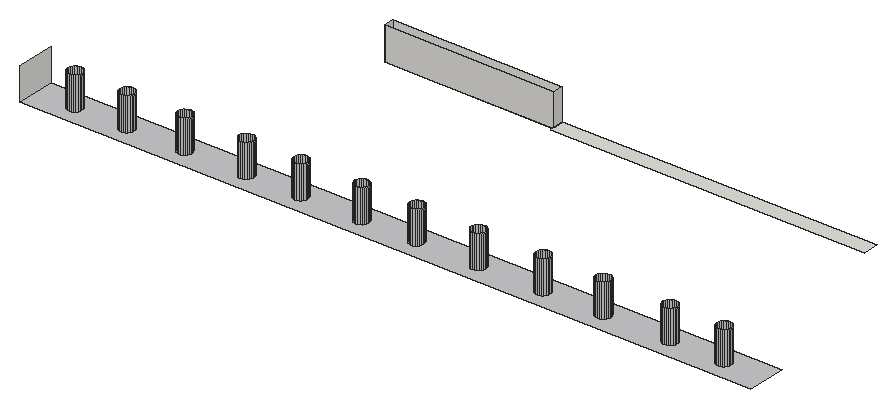
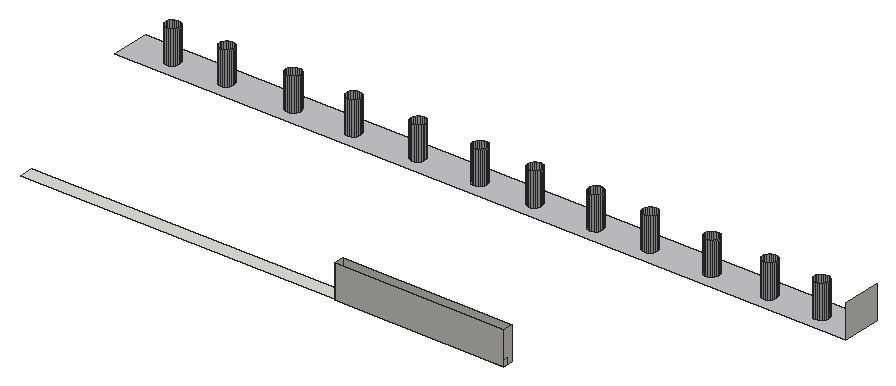
# SketchUp Ruby script. Lengths in inches.
U = 1.inch
M = Sketchup.active_model
def pt(a) = Geom::Point3d.new(a.map { |v| v * U })
def face(e, loops, mat)
  f = e.add_face(loops[0].map { |a| pt(a) })
  loops[1..].each { |l| e.add_face(l.map { |a| pt(a) }).erase! }
  f.material = f.back_material = mat if mat
  f
end
# faces: each face lists its corners as indices into pts; further lists are holes
def faces(e, pts, list, mat = nil) = list.each { |f| face(e, (f[0].is_a?(Array) ? f : [f]).map { |l| l.map { |i| pts[i] } }, mat) }
# xy, xz, yz: faces in a plane at the given z, y or x. An outline is a flat list of corners, or four numbers for a rectangle; further outlines are holes
def ring(l) = l.size == 4 ? [[l[0], l[1]], [l[2], l[1]], [l[2], l[3]], [l[0], l[3]]] : l.each_slice(2).to_a
def flat(e, list, mat, &to3) = list.each { |f| face(e, (f[0].is_a?(Array) ? f : [f]).map { |l| ring(l).map { |u, v| to3.(u, v) } }, mat) }
def xy(e, z, list, mat = nil) = flat(e, list, mat) { |x, y| [x, y, z] }
def xz(e, y, list, mat = nil) = flat(e, list, mat) { |x, z| [x, y, z] }
def yz(e, x, list, mat = nil) = flat(e, list, mat) { |y, z| [x, y, z] }
def lines(e, pts, list) = list.each { |a, b| e.add_line(pt(pts[a]), pt(pts[b])) }
# prism: a flat outline (further loops are holes) pulled along v
def prism(e, loops, v, mat = nil)
  f = face(e, loops, mat); d = Geom::Vector3d.new(v.map { |x| x * U })
  f.pushpull(f.normal.samedirection?(d) ? d.length : -d.length)
end
def box(e, o, s, mat = nil) = prism(e, [[o, [o[0] + s[0], o[1], o[2]], [o[0] + s[0], o[1] + s[1], o[2]], [o[0], o[1] + s[1], o[2]]]], [0, 0, s[2]], mat)
def at(x, y, z, deg = 0) = Geom::Transformation.translation(pt([x, y, z])) * Geom::Transformation.rotation(ORIGIN, Z_AXIS, deg.degrees)
def axes(o, x, y, z) = Geom::Transformation.new([*x, 0, *y, 0, *z, 0, *pt(o).to_a, 1])
def part(name) = M.definitions.add(name)
# library, detail: a bought-in or finely detailed component or shape, given as its bounding box
def library(name, o, s) = part(name).tap { |d| box(d.entities, o, s) }
def detail(e, o, s) = box(e.add_group.entities, o, s)
def put(e, d, t, mat = nil) = e.add_instance(d, t).tap { |i| i.material = mat if mat }
def group(e, t, mat = nil) = e.add_group.tap { |g| g.transformation = t; g.material = mat if mat }.entities
root = M.entities
M.materials.add("[Polished Concrete New]").color = [200, 200, 203]
M.materials.add("[Terrazzo Tile Accent]").color = [224, 221, 217]
xy(root,116.26,[[461.1,311.53,526.2,315.41]],"[Terrazzo Tile Accent]")
xy(root,116.34,[[406,228.82,405.29,228.92,404.625,229.19,404.06,229.63,403.62,230.2,403.34,230.86,403.25,231.57,403.34,232.29,403.62,232.95,404.06,233.52,404.625,233.96,405.29,234.23,406,234.32,406.71,234.23,407.375,233.96,407.94,233.52,408.38,232.95,408.66,232.29,408.75,231.57,408.66,230.86,408.38,230.2,407.94,229.63,407.375,229.19,406.71,228.92],[426,228.82,425.29,228.92,424.625,229.19,424.06,229.63,423.62,230.2,423.34,230.86,423.25,231.57,423.34,232.29,423.62,232.95,424.06,233.52,424.625,233.96,425.29,234.23,426,234.32,426.71,234.23,427.375,233.96,427.94,233.52,428.38,232.95,428.66,232.29,428.75,231.57,428.66,230.86,428.38,230.2,427.94,229.63,427.375,229.19,426.71,228.92],[448.1875,228.82,447.48,228.92,446.8125,229.19,446.24,229.63,445.81,230.2,445.53,230.86,445.4375,231.57,445.53,232.29,445.81,232.95,446.24,233.52,446.8125,233.96,447.48,234.23,448.1875,234.32,448.9,234.23,449.5625,233.96,450.13,233.52,450.57,232.95,450.84,232.29,450.9375,231.57,450.84,230.86,450.57,230.2,450.13,229.63,449.5625,229.19,448.9,228.92],[471.875,228.82,471.16,228.92,470.5,229.19,469.93,229.63,469.49,230.2,469.22,230.86,469.125,231.57,469.22,232.29,469.49,232.95,469.93,233.52,470.5,233.96,471.16,234.23,471.875,234.32,472.59,234.23,473.25,233.96,473.82,233.52,474.26,232.95,474.53,232.29,474.625,231.57,474.53,230.86,474.26,230.2,473.82,229.63,473.25,229.19,472.59,228.92],[492.8125,228.82,492.1,228.92,491.4375,229.19,490.87,229.63,490.43,230.2,490.16,230.86,490.0625,231.57,490.16,232.29,490.43,232.95,490.87,233.52,491.4375,233.96,492.1,234.23,492.8125,234.32,493.52,234.23,494.1875,233.96,494.76,233.52,495.19,232.95,495.47,232.29,495.5625,231.57,495.47,230.86,495.19,230.2,494.76,229.63,494.1875,229.19,493.52,228.92],
  [516.1875,228.82,515.48,228.92,514.8125,229.19,514.24,229.63,513.81,230.2,513.53,230.86,513.4375,231.57,513.53,232.29,513.81,232.95,514.24,233.52,514.8125,233.96,515.48,234.23,516.1875,234.32,516.9,234.23,517.5625,233.96,518.13,233.52,518.57,232.95,518.84,232.29,518.9375,231.57,518.84,230.86,518.57,230.2,518.13,229.63,517.5625,229.19,516.9,228.92],[537.375,228.82,536.66,228.92,536,229.19,535.43,229.63,534.99,230.2,534.72,230.86,534.625,231.57,534.72,232.29,534.99,232.95,535.43,233.52,536,233.96,536.66,234.23,537.375,234.32,538.09,234.23,538.75,233.96,539.32,233.52,539.76,232.95,540.03,232.29,540.125,231.57,540.03,230.86,539.76,230.2,539.32,229.63,538.75,229.19,538.09,228.92],[561.125,228.82,560.41,228.92,559.75,229.19,559.18,229.63,558.74,230.2,558.47,230.86,558.375,231.57,558.47,232.29,558.74,232.95,559.18,233.52,559.75,233.96,560.41,234.23,561.125,234.32,561.84,234.23,562.5,233.96,563.07,233.52,563.51,232.95,563.78,232.29,563.875,231.57,563.78,230.86,563.51,230.2,563.07,229.63,562.5,229.19,561.84,228.92],[585.9375,228.82,585.23,228.92,584.5625,229.19,583.99,229.63,583.56,230.2,583.28,230.86,583.1875,231.57,583.28,232.29,583.56,232.95,583.99,233.52,584.5625,233.96,585.23,234.23,585.9375,234.32,586.65,234.23,587.3125,233.96,587.88,233.52,588.32,232.95,588.59,232.29,588.6875,231.57,588.59,230.86,588.32,230.2,587.88,229.63,587.3125,229.19,586.65,228.92],[609.0625,228.82,608.35,228.92,607.6875,229.19,607.12,229.63,606.68,230.2,606.41,230.86,606.3125,231.57,606.41,232.29,606.68,232.95,607.12,233.52,607.6875,233.96,608.35,234.23,609.0625,234.32,609.77,234.23,610.4375,233.96,611.01,233.52,611.44,232.95,611.72,232.29,611.8125,231.57,611.72,230.86,611.44,230.2,611.01,229.63,610.4375,229.19,609.77,228.92],
  [634.75,228.82,634.04,228.92,633.375,229.19,632.81,229.63,632.37,230.2,632.09,230.86,632,231.57,632.09,232.29,632.37,232.95,632.81,233.52,633.375,233.96,634.04,234.23,634.75,234.32,635.46,234.23,636.125,233.96,636.69,233.52,637.13,232.95,637.41,232.29,637.5,231.57,637.41,230.86,637.13,230.2,636.69,229.63,636.125,229.19,635.46,228.92],[655.5,228.82,654.79,228.92,654.125,229.19,653.56,229.63,653.12,230.2,652.84,230.86,652.75,231.57,652.84,232.29,653.12,232.95,653.56,233.52,654.125,233.96,654.79,234.23,655.5,234.32,656.21,234.23,656.875,233.96,657.44,233.52,657.88,232.95,658.16,232.29,658.25,231.57,658.16,230.86,657.88,230.2,657.44,229.63,656.875,229.19,656.21,228.92]])
xy(root,116.34,[[[391.12,223.85,671.95,238.73],[655.5,228.82,654.79,228.92,654.125,229.19,653.56,229.63,653.12,230.2,652.84,230.86,652.75,231.57,652.84,232.29,653.12,232.95,653.56,233.52,654.125,233.96,654.79,234.23,655.5,234.32,656.21,234.23,656.875,233.96,657.44,233.52,657.88,232.95,658.16,232.29,658.25,231.57,658.16,230.86,657.88,230.2,657.44,229.63,656.875,229.19,656.21,228.92],[426,228.82,425.29,228.92,424.625,229.19,424.06,229.63,423.62,230.2,423.34,230.86,423.25,231.57,423.34,232.29,423.62,232.95,424.06,233.52,424.625,233.96,425.29,234.23,426,234.32,426.71,234.23,427.375,233.96,427.94,233.52,428.38,232.95,428.66,232.29,428.75,231.57,428.66,230.86,428.38,230.2,427.94,229.63,427.375,229.19,426.71,228.92],[634.75,228.82,634.04,228.92,633.375,229.19,632.81,229.63,632.37,230.2,632.09,230.86,632,231.57,632.09,232.29,632.37,232.95,632.81,233.52,633.375,233.96,634.04,234.23,634.75,234.32,635.46,234.23,636.125,233.96,636.69,233.52,637.13,232.95,637.41,232.29,637.5,231.57,637.41,230.86,637.13,230.2,636.69,229.63,636.125,229.19,635.46,228.92],[448.1875,228.82,447.48,228.92,446.8125,229.19,446.24,229.63,445.81,230.2,445.53,230.86,445.4375,231.57,445.53,232.29,445.81,232.95,446.24,233.52,446.8125,233.96,447.48,234.23,448.1875,234.32,448.9,234.23,449.5625,233.96,450.13,233.52,450.57,232.95,450.84,232.29,450.9375,231.57,450.84,230.86,450.57,230.2,450.13,229.63,449.5625,229.19,448.9,228.92],[609.0625,228.82,608.35,228.92,607.6875,229.19,607.12,229.63,606.68,230.2,606.41,230.86,606.3125,231.57,606.41,232.29,606.68,232.95,607.12,233.52,607.6875,233.96,608.35,234.23,609.0625,234.32,609.77,234.23,610.4375,233.96,611.01,233.52,611.44,232.95,611.72,232.29,611.8125,231.57,611.72,230.86,611.44,230.2,611.01,229.63,610.4375,229.19,609.77,228.92],[471.875,228.82,471.16,228.92,470.5,229.19,469.93,229.63,469.49,230.2,469.22,230.86,469.125,231.57,469.22,232.29,469.49,232.95,469.93,233.52,470.5,233.96,471.16,234.23,471.875,234.32,472.59,234.23,473.25,233.96,473.82,233.52,474.26,232.95,474.53,232.29,474.625,231.57,474.53,230.86,474.26,230.2,473.82,229.63,473.25,229.19,472.59,228.92],[585.9375,228.82,585.23,228.92,584.5625,229.19,583.99,229.63,583.56,230.2,583.28,230.86,583.1875,231.57,583.28,232.29,583.56,232.95,583.99,233.52,584.5625,233.96,585.23,234.23,585.9375,234.32,586.65,234.23,587.3125,233.96,587.88,233.52,588.32,232.95,588.59,232.29,588.6875,231.57,588.59,230.86,588.32,230.2,587.88,229.63,587.3125,229.19,586.65,228.92],[492.8125,228.82,492.1,228.92,491.4375,229.19,490.87,229.63,490.43,230.2,490.16,230.86,490.0625,231.57,490.16,232.29,490.43,232.95,490.87,233.52,491.4375,233.96,492.1,234.23,492.8125,234.32,493.52,234.23,494.1875,233.96,494.76,233.52,495.19,232.95,495.47,232.29,495.5625,231.57,495.47,230.86,495.19,230.2,494.76,229.63,494.1875,229.19,493.52,228.92],[561.125,228.82,560.41,228.92,559.75,229.19,559.18,229.63,558.74,230.2,558.47,230.86,558.375,231.57,558.47,232.29,558.74,232.95,559.18,233.52,559.75,233.96,560.41,234.23,561.125,234.32,561.84,234.23,562.5,233.96,563.07,233.52,563.51,232.95,563.78,232.29,563.875,231.57,563.78,230.86,563.51,230.2,563.07,229.63,562.5,229.19,561.84,228.92],[516.1875,228.82,515.48,228.92,514.8125,229.19,514.24,229.63,513.81,230.2,513.53,230.86,513.4375,231.57,513.53,232.29,513.81,232.95,514.24,233.52,514.8125,233.96,515.48,234.23,516.1875,234.32,516.9,234.23,517.5625,233.96,518.13,233.52,518.57,232.95,518.84,232.29,518.9375,231.57,518.84,230.86,518.57,230.2,518.13,229.63,517.5625,229.19,516.9,228.92],[537.375,228.82,536.66,228.92,536,229.19,535.43,229.63,534.99,230.2,534.72,230.86,534.625,231.57,534.72,232.29,534.99,232.95,535.43,233.52,536,233.96,536.66,234.23,537.375,234.32,538.09,234.23,538.75,233.96,539.32,233.52,539.76,232.95,540.03,232.29,540.125,231.57,540.03,230.86,539.76,230.2,539.32,229.63,538.75,229.19,538.09,228.92],[406,228.82,405.29,228.92,404.625,229.19,404.06,229.63,403.62,230.2,403.34,230.86,403.25,231.57,403.34,232.29,403.62,232.95,404.06,233.52,404.625,233.96,405.29,234.23,406,234.32,406.71,234.23,407.375,233.96,407.94,233.52,408.38,232.95,408.66,232.29,408.75,231.57,408.66,230.86,408.38,230.2,407.94,229.63,407.375,229.19,406.71,228.92]]],"[Polished Concrete New]")
xy(root,116.71,[[526.2,309.72,646.95,315.41]])
xz(root,311.53,[[461.1,116.26,526.2,129]],"[Terrazzo Tile Accent]")
xz(root,315.41,[[461.1,116.26,526.2,129]])
yz(root,391.12,[[223.85,116.34,238.73,129]])
yz(root,461.1,[[313.78,116.26,315.41,118.57]])
yz(root,461.1,[[311.53,116.26,311.53,129,315.41,129,315.41,118.57,313.78,118.57,313.78,116.26]],"[Terrazzo Tile Accent]")
yz(root,526.2,[[311.53,116.26,315.41,116.71]])
yz(root,526.2,[[311.53,116.71,315.41,129]],"[Terrazzo Tile Accent]")
p = [[405.29,228.92,116.34],[406,228.82,116.34],[406,228.82,129],[405.29,228.92,129],[406.71,228.92,116.34],[406.71,228.92,129],
  [425.29,228.92,116.34],[426,228.82,116.34],[426,228.82,129],[425.29,228.92,129],[426.71,228.92,116.34],[426.71,228.92,129],
  [447.48,228.92,116.34],[448.1875,228.82,116.34],[448.1875,228.82,129],[447.48,228.92,129],[448.9,228.92,116.34],[448.9,228.92,129],
  [471.16,228.92,116.34],[471.875,228.82,116.34],[471.875,228.82,129],[471.16,228.92,129],[472.59,228.92,116.34],[472.59,228.92,129],
  [492.1,228.92,116.34],[492.8125,228.82,116.34],[492.8125,228.82,129],[492.1,228.92,129],[493.52,228.92,116.34],[493.52,228.92,129],
  [515.48,228.92,116.34],[516.1875,228.82,116.34],[516.1875,228.82,129],[515.48,228.92,129],[516.9,228.92,116.34],[516.9,228.92,129],
  [536.66,228.92,116.34],[537.375,228.82,116.34],[537.375,228.82,129],[536.66,228.92,129],[538.09,228.92,116.34],[538.09,228.92,129],
  [560.41,228.92,116.34],[561.125,228.82,116.34],[561.125,228.82,129],[560.41,228.92,129],[561.84,228.92,116.34],[561.84,228.92,129],
  [585.23,228.92,116.34],[585.9375,228.82,116.34],[585.9375,228.82,129],[585.23,228.92,129],[586.65,228.92,116.34],[586.65,228.92,129],
  [608.35,228.92,116.34],[609.0625,228.82,116.34],[609.0625,228.82,129],[608.35,228.92,129],[609.77,228.92,116.34],[609.77,228.92,129],
  [634.04,228.92,116.34],[634.75,228.82,116.34],[634.75,228.82,129],[634.04,228.92,129],[635.46,228.92,116.34],[635.46,228.92,129],
  [654.79,228.92,116.34],[655.5,228.82,116.34],[655.5,228.82,129],[654.79,228.92,129],[656.21,228.92,116.34],[656.21,228.92,129],
  [404.625,229.19,116.34],[404.625,229.19,129],[407.375,229.19,116.34],[407.375,229.19,129],[424.625,229.19,116.34],[424.625,229.19,129],
  [427.375,229.19,116.34],[427.375,229.19,129],[446.8125,229.19,116.34],[446.8125,229.19,129],[449.5625,229.19,116.34],[449.5625,229.19,129],
  [470.5,229.19,116.34],[470.5,229.19,129],[473.25,229.19,116.34],[473.25,229.19,129],[491.4375,229.19,116.34],[491.4375,229.19,129],
  [494.1875,229.19,116.34],[494.1875,229.19,129],[514.8125,229.19,116.34],[514.8125,229.19,129],[517.5625,229.19,116.34],[517.5625,229.19,129],
  [536,229.19,116.34],[536,229.19,129],[538.75,229.19,116.34],[538.75,229.19,129],[559.75,229.19,116.34],[559.75,229.19,129],
  [562.5,229.19,116.34],[562.5,229.19,129],[584.5625,229.19,116.34],[584.5625,229.19,129],[587.3125,229.19,116.34],[587.3125,229.19,129],
  [607.6875,229.19,116.34],[607.6875,229.19,129],[610.4375,229.19,116.34],[610.4375,229.19,129],[633.375,229.19,116.34],[633.375,229.19,129],
  [636.125,229.19,116.34],[636.125,229.19,129],[654.125,229.19,116.34],[654.125,229.19,129],[656.875,229.19,116.34],[656.875,229.19,129],
  [404.06,229.63,116.34],[404.06,229.63,129],[407.94,229.63,116.34],[407.94,229.63,129],[424.06,229.63,116.34],[424.06,229.63,129],
  [427.94,229.63,116.34],[427.94,229.63,129],[446.24,229.63,116.34],[446.24,229.63,129],[450.13,229.63,116.34],[450.13,229.63,129],
  [469.93,229.63,116.34],[469.93,229.63,129],[473.82,229.63,116.34],[473.82,229.63,129],[490.87,229.63,116.34],[490.87,229.63,129],
  [494.76,229.63,116.34],[494.76,229.63,129],[514.24,229.63,116.34],[514.24,229.63,129],[518.13,229.63,116.34],[518.13,229.63,129],
  [535.43,229.63,116.34],[535.43,229.63,129],[539.32,229.63,116.34],[539.32,229.63,129],[559.18,229.63,116.34],[559.18,229.63,129],
  [563.07,229.63,116.34],[563.07,229.63,129],[583.99,229.63,116.34],[583.99,229.63,129],[587.88,229.63,116.34],[587.88,229.63,129],
  [607.12,229.63,116.34],[607.12,229.63,129],[611.01,229.63,116.34],[611.01,229.63,129],[632.81,229.63,116.34],[632.81,229.63,129],
  [636.69,229.63,116.34],[636.69,229.63,129],[653.56,229.63,116.34],[653.56,229.63,129],[657.44,229.63,116.34],[657.44,229.63,129],
  [403.62,230.2,116.34],[403.62,230.2,129],[408.38,230.2,116.34],[408.38,230.2,129],[423.62,230.2,116.34],[423.62,230.2,129],
  [428.38,230.2,116.34],[428.38,230.2,129],[445.81,230.2,116.34],[445.81,230.2,129],[450.57,230.2,116.34],[450.57,230.2,129],
  [469.49,230.2,116.34],[469.49,230.2,129],[474.26,230.2,116.34],[474.26,230.2,129],[490.43,230.2,116.34],[490.43,230.2,129],
  [495.19,230.2,116.34],[495.19,230.2,129],[513.81,230.2,116.34],[513.81,230.2,129],[518.57,230.2,116.34],[518.57,230.2,129],
  [534.99,230.2,116.34],[534.99,230.2,129],[539.76,230.2,116.34],[539.76,230.2,129],[558.74,230.2,116.34],[558.74,230.2,129],
  [563.51,230.2,116.34],[563.51,230.2,129],[583.56,230.2,116.34],[583.56,230.2,129],[588.32,230.2,116.34],[588.32,230.2,129],
  [606.68,230.2,116.34],[606.68,230.2,129],[611.44,230.2,116.34],[611.44,230.2,129],[632.37,230.2,116.34],[632.37,230.2,129],
  [637.13,230.2,116.34],[637.13,230.2,129],[653.12,230.2,116.34],[653.12,230.2,129],[657.88,230.2,116.34],[657.88,230.2,129],
  [403.34,230.86,116.34],[403.34,230.86,129],[408.66,230.86,116.34],[408.66,230.86,129],[423.34,230.86,116.34],[423.34,230.86,129],
  [428.66,230.86,116.34],[428.66,230.86,129],[445.53,230.86,116.34],[445.53,230.86,129],[450.84,230.86,116.34],[450.84,230.86,129],
  [469.22,230.86,116.34],[469.22,230.86,129],[474.53,230.86,116.34],[474.53,230.86,129],[490.16,230.86,116.34],[490.16,230.86,129],
  [495.47,230.86,116.34],[495.47,230.86,129],[513.53,230.86,116.34],[513.53,230.86,129],[518.84,230.86,116.34],[518.84,230.86,129],
  [534.72,230.86,116.34],[534.72,230.86,129],[540.03,230.86,116.34],[540.03,230.86,129],[558.47,230.86,116.34],[558.47,230.86,129],
  [563.78,230.86,116.34],[563.78,230.86,129],[583.28,230.86,116.34],[583.28,230.86,129],[588.59,230.86,116.34],[588.59,230.86,129],
  [606.41,230.86,116.34],[606.41,230.86,129],[611.72,230.86,116.34],[611.72,230.86,129],[632.09,230.86,116.34],[632.09,230.86,129],
  [637.41,230.86,116.34],[637.41,230.86,129],[652.84,230.86,116.34],[652.84,230.86,129],[658.16,230.86,116.34],[658.16,230.86,129],
  [403.25,231.57,116.34],[403.25,231.57,129],[408.75,231.57,116.34],[408.75,231.57,129],[423.25,231.57,116.34],[423.25,231.57,129],
  [428.75,231.57,116.34],[428.75,231.57,129],[445.4375,231.57,116.34],[445.4375,231.57,129],[450.9375,231.57,116.34],[450.9375,231.57,129],
  [469.125,231.57,116.34],[469.125,231.57,129],[474.625,231.57,116.34],[474.625,231.57,129],[490.0625,231.57,116.34],[490.0625,231.57,129],
  [495.5625,231.57,116.34],[495.5625,231.57,129],[513.4375,231.57,116.34],[513.4375,231.57,129],[518.9375,231.57,116.34],[518.9375,231.57,129],
  [534.625,231.57,116.34],[534.625,231.57,129],[540.125,231.57,116.34],[540.125,231.57,129],[558.375,231.57,116.34],[558.375,231.57,129],
  [563.875,231.57,116.34],[563.875,231.57,129],[583.1875,231.57,116.34],[583.1875,231.57,129],[588.6875,231.57,116.34],[588.6875,231.57,129],
  [606.3125,231.57,116.34],[606.3125,231.57,129],[611.8125,231.57,116.34],[611.8125,231.57,129],[632,231.57,116.34],[632,231.57,129],
  [637.5,231.57,116.34],[637.5,231.57,129],[652.75,231.57,116.34],[652.75,231.57,129],[658.25,231.57,116.34],[658.25,231.57,129],
  [403.34,232.29,116.34],[403.34,232.29,129],[408.66,232.29,116.34],[408.66,232.29,129],[423.34,232.29,116.34],[423.34,232.29,129],
  [428.66,232.29,116.34],[428.66,232.29,129],[445.53,232.29,116.34],[445.53,232.29,129],[450.84,232.29,116.34],[450.84,232.29,129],
  [469.22,232.29,116.34],[469.22,232.29,129],[474.53,232.29,116.34],[474.53,232.29,129],[490.16,232.29,116.34],[490.16,232.29,129],
  [495.47,232.29,116.34],[495.47,232.29,129],[513.53,232.29,116.34],[513.53,232.29,129],[518.84,232.29,116.34],[518.84,232.29,129],
  [534.72,232.29,116.34],[534.72,232.29,129],[540.03,232.29,116.34],[540.03,232.29,129],[558.47,232.29,116.34],[558.47,232.29,129],
  [563.78,232.29,116.34],[563.78,232.29,129],[583.28,232.29,116.34],[583.28,232.29,129],[588.59,232.29,116.34],[588.59,232.29,129],
  [606.41,232.29,116.34],[606.41,232.29,129],[611.72,232.29,116.34],[611.72,232.29,129],[632.09,232.29,116.34],[632.09,232.29,129],
  [637.41,232.29,116.34],[637.41,232.29,129],[652.84,232.29,116.34],[652.84,232.29,129],[658.16,232.29,116.34],[658.16,232.29,129],
  [403.62,232.95,116.34],[403.62,232.95,129],[408.38,232.95,116.34],[408.38,232.95,129],[423.62,232.95,116.34],[423.62,232.95,129],
  [428.38,232.95,116.34],[428.38,232.95,129],[445.81,232.95,116.34],[445.81,232.95,129],[450.57,232.95,116.34],[450.57,232.95,129],
  [469.49,232.95,116.34],[469.49,232.95,129],[474.26,232.95,116.34],[474.26,232.95,129],[490.43,232.95,116.34],[490.43,232.95,129],
  [495.19,232.95,116.34],[495.19,232.95,129],[513.81,232.95,116.34],[513.81,232.95,129],[518.57,232.95,116.34],[518.57,232.95,129],
  [534.99,232.95,116.34],[534.99,232.95,129],[539.76,232.95,116.34],[539.76,232.95,129],[558.74,232.95,116.34],[558.74,232.95,129],
  [563.51,232.95,116.34],[563.51,232.95,129],[583.56,232.95,116.34],[583.56,232.95,129],[588.32,232.95,116.34],[588.32,232.95,129],
  [606.68,232.95,116.34],[606.68,232.95,129],[611.44,232.95,116.34],[611.44,232.95,129],[632.37,232.95,116.34],[632.37,232.95,129],
  [637.13,232.95,116.34],[637.13,232.95,129],[653.12,232.95,116.34],[653.12,232.95,129],[657.88,232.95,116.34],[657.88,232.95,129],
  [404.06,233.52,116.34],[404.06,233.52,129],[407.94,233.52,116.34],[407.94,233.52,129],[424.06,233.52,116.34],[424.06,233.52,129],
  [427.94,233.52,116.34],[427.94,233.52,129],[446.24,233.52,116.34],[446.24,233.52,129],[450.13,233.52,116.34],[450.13,233.52,129],
  [469.93,233.52,116.34],[469.93,233.52,129],[473.82,233.52,116.34],[473.82,233.52,129],[490.87,233.52,116.34],[490.87,233.52,129],
  [494.76,233.52,116.34],[494.76,233.52,129],[514.24,233.52,116.34],[514.24,233.52,129],[518.13,233.52,116.34],[518.13,233.52,129],
  [535.43,233.52,116.34],[535.43,233.52,129],[539.32,233.52,116.34],[539.32,233.52,129],[559.18,233.52,116.34],[559.18,233.52,129],
  [563.07,233.52,116.34],[563.07,233.52,129],[583.99,233.52,116.34],[583.99,233.52,129],[587.88,233.52,116.34],[587.88,233.52,129],
  [607.12,233.52,116.34],[607.12,233.52,129],[611.01,233.52,116.34],[611.01,233.52,129],[632.81,233.52,116.34],[632.81,233.52,129],
  [636.69,233.52,116.34],[636.69,233.52,129],[653.56,233.52,116.34],[653.56,233.52,129],[657.44,233.52,116.34],[657.44,233.52,129],
  [404.625,233.96,116.34],[404.625,233.96,129],[407.375,233.96,116.34],[407.375,233.96,129],[424.625,233.96,116.34],[424.625,233.96,129],
  [427.375,233.96,116.34],[427.375,233.96,129],[446.8125,233.96,116.34],[446.8125,233.96,129],[449.5625,233.96,116.34],[449.5625,233.96,129],
  [470.5,233.96,116.34],[470.5,233.96,129],[473.25,233.96,116.34],[473.25,233.96,129],[491.4375,233.96,116.34],[491.4375,233.96,129],
  [494.1875,233.96,116.34],[494.1875,233.96,129],[514.8125,233.96,116.34],[514.8125,233.96,129],[517.5625,233.96,116.34],[517.5625,233.96,129],
  [536,233.96,116.34],[536,233.96,129],[538.75,233.96,116.34],[538.75,233.96,129],[559.75,233.96,116.34],[559.75,233.96,129],
  [562.5,233.96,116.34],[562.5,233.96,129],[584.5625,233.96,116.34],[584.5625,233.96,129],[587.3125,233.96,116.34],[587.3125,233.96,129],
  [607.6875,233.96,116.34],[607.6875,233.96,129],[610.4375,233.96,116.34],[610.4375,233.96,129],[633.375,233.96,116.34],[633.375,233.96,129],
  [636.125,233.96,116.34],[636.125,233.96,129],[654.125,233.96,116.34],[654.125,233.96,129],[656.875,233.96,116.34],[656.875,233.96,129],
  [405.29,234.23,116.34],[405.29,234.23,129],[406.71,234.23,116.34],[406.71,234.23,129],[425.29,234.23,116.34],[425.29,234.23,129],
  [426.71,234.23,116.34],[426.71,234.23,129],[447.48,234.23,116.34],[447.48,234.23,129],[448.9,234.23,116.34],[448.9,234.23,129],
  [471.16,234.23,116.34],[471.16,234.23,129],[472.59,234.23,116.34],[472.59,234.23,129],[492.1,234.23,116.34],[492.1,234.23,129],
  [493.52,234.23,116.34],[493.52,234.23,129],[515.48,234.23,116.34],[515.48,234.23,129],[516.9,234.23,116.34],[516.9,234.23,129],
  [536.66,234.23,116.34],[536.66,234.23,129],[538.09,234.23,116.34],[538.09,234.23,129],[560.41,234.23,116.34],[560.41,234.23,129],
  [561.84,234.23,116.34],[561.84,234.23,129],[585.23,234.23,116.34],[585.23,234.23,129],[586.65,234.23,116.34],[586.65,234.23,129],
  [608.35,234.23,116.34],[608.35,234.23,129],[609.77,234.23,116.34],[609.77,234.23,129],[634.04,234.23,116.34],[634.04,234.23,129],
  [635.46,234.23,116.34],[635.46,234.23,129],[654.79,234.23,116.34],[654.79,234.23,129],[656.21,234.23,116.34],[656.21,234.23,129],
  [406,234.32,116.34],[406,234.32,129],[426,234.32,116.34],[426,234.32,129],[448.1875,234.32,116.34],[448.1875,234.32,129],
  [471.875,234.32,116.34],[471.875,234.32,129],[492.8125,234.32,116.34],[492.8125,234.32,129],[516.1875,234.32,116.34],[516.1875,234.32,129],
  [537.375,234.32,116.34],[537.375,234.32,129],[561.125,234.32,116.34],[561.125,234.32,129],[585.9375,234.32,116.34],[585.9375,234.32,129],
  [609.0625,234.32,116.34],[609.0625,234.32,129],[634.75,234.32,116.34],[634.75,234.32,129],[655.5,234.32,116.34],[655.5,234.32,129]]
faces(root,p,[[0,1,2,3],[1,4,5,2],[6,7,8,9],[7,10,11,8],[12,13,14,15],[13,16,17,14],[18,19,20,21],[19,22,23,20],
  [24,25,26,27],[25,28,29,26],[30,31,32,33],[31,34,35,32],[36,37,38,39],[37,40,41,38],[42,43,44,45],[43,46,47,44],
  [48,49,50,51],[49,52,53,50],[54,55,56,57],[55,58,59,56],[60,61,62,63],[61,64,65,62],[66,67,68,69],[67,70,71,68],
  [72,0,3,73],[4,74,75,5],[76,6,9,77],[10,78,79,11],[80,12,15,81],[16,82,83,17],[84,18,21,85],[22,86,87,23],
  [88,24,27,89],[28,90,91,29],[92,30,33,93],[34,94,95,35],[96,36,39,97],[40,98,99,41],[100,42,45,101],[46,102,103,47],
  [104,48,51,105],[52,106,107,53],[108,54,57,109],[58,110,111,59],[112,60,63,113],[64,114,115,65],[116,66,69,117],[70,118,119,71],
  [120,72,73,121],[74,122,123,75],[124,76,77,125],[78,126,127,79],[128,80,81,129],[82,130,131,83],[132,84,85,133],[86,134,135,87],
  [136,88,89,137],[90,138,139,91],[140,92,93,141],[94,142,143,95],[144,96,97,145],[98,146,147,99],[148,100,101,149],[102,150,151,103],
  [152,104,105,153],[106,154,155,107],[156,108,109,157],[110,158,159,111],[160,112,113,161],[114,162,163,115],[164,116,117,165],[118,166,167,119],
  [168,120,121,169],[122,170,171,123],[172,124,125,173],[126,174,175,127],[176,128,129,177],[130,178,179,131],[180,132,133,181],[134,182,183,135],
  [184,136,137,185],[138,186,187,139],[188,140,141,189],[142,190,191,143],[192,144,145,193],[146,194,195,147],[196,148,149,197],[150,198,199,151],
  [200,152,153,201],[154,202,203,155],[204,156,157,205],[158,206,207,159],[208,160,161,209],[162,210,211,163],[212,164,165,213],[166,214,215,167],
  [216,168,169,217],[170,218,219,171],[220,172,173,221],[174,222,223,175],[224,176,177,225],[178,226,227,179],[228,180,181,229],[182,230,231,183],
  [232,184,185,233],[186,234,235,187],[236,188,189,237],[190,238,239,191],[240,192,193,241],[194,242,243,195],[244,196,197,245],[198,246,247,199],
  [248,200,201,249],[202,250,251,203],[252,204,205,253],[206,254,255,207],[256,208,209,257],[210,258,259,211],[260,212,213,261],[214,262,263,215],
  [264,216,217,265],[218,266,267,219],[268,220,221,269],[222,270,271,223],[272,224,225,273],[226,274,275,227],[276,228,229,277],[230,278,279,231],
  [280,232,233,281],[234,282,283,235],[284,236,237,285],[238,286,287,239],[288,240,241,289],[242,290,291,243],[292,244,245,293],[246,294,295,247],
  [296,248,249,297],[250,298,299,251],[300,252,253,301],[254,302,303,255],[304,256,257,305],[258,306,307,259],[308,260,261,309],[262,310,311,263],
  [312,264,265,313],[266,314,315,267],[316,268,269,317],[270,318,319,271],[320,272,273,321],[274,322,323,275],[324,276,277,325],[278,326,327,279],
  [328,280,281,329],[282,330,331,283],[332,284,285,333],[286,334,335,287],[336,288,289,337],[290,338,339,291],[340,292,293,341],[294,342,343,295],
  [344,296,297,345],[298,346,347,299],[348,300,301,349],[302,350,351,303],[352,304,305,353],[306,354,355,307],[356,308,309,357],[310,358,359,311],
  [360,312,313,361],[314,362,363,315],[364,316,317,365],[318,366,367,319],[368,320,321,369],[322,370,371,323],[372,324,325,373],[326,374,375,327],
  [376,328,329,377],[330,378,379,331],[380,332,333,381],[334,382,383,335],[384,336,337,385],[338,386,387,339],[388,340,341,389],[342,390,391,343],
  [392,344,345,393],[346,394,395,347],[396,348,349,397],[350,398,399,351],[400,352,353,401],[354,402,403,355],[404,356,357,405],[358,406,407,359],
  [408,360,361,409],[362,410,411,363],[412,364,365,413],[366,414,415,367],[416,368,369,417],[370,418,419,371],[420,372,373,421],[374,422,423,375],
  [424,376,377,425],[378,426,427,379],[428,380,381,429],[382,430,431,383],[432,384,385,433],[386,434,435,387],[436,388,389,437],[390,438,439,391],
  [440,392,393,441],[394,442,443,395],[444,396,397,445],[398,446,447,399],[448,400,401,449],[402,450,451,403],[452,404,405,453],[406,454,455,407],
  [456,408,409,457],[410,458,459,411],[460,412,413,461],[414,462,463,415],[464,416,417,465],[418,466,467,419],[468,420,421,469],[422,470,471,423],
  [472,424,425,473],[426,474,475,427],[476,428,429,477],[430,478,479,431],[480,432,433,481],[434,482,483,435],[484,436,437,485],[438,486,487,439],
  [488,440,441,489],[442,490,491,443],[492,444,445,493],[446,494,495,447],[496,448,449,497],[450,498,499,451],[500,452,453,501],[454,502,503,455],
  [504,456,457,505],[458,506,507,459],[508,460,461,509],[462,510,511,463],[512,464,465,513],[466,514,515,467],[516,468,469,517],[470,518,519,471],
  [520,472,473,521],[474,522,523,475],[524,476,477,525],[478,526,527,479],[528,480,481,529],[482,530,531,483],[532,484,485,533],[486,534,535,487],
  [536,488,489,537],[490,538,539,491],[540,492,493,541],[494,542,543,495],[544,496,497,545],[498,546,547,499],[548,500,501,549],[502,550,551,503],
  [552,504,505,553],[506,552,553,507],[554,508,509,555],[510,554,555,511],[556,512,513,557],[514,556,557,515],[558,516,517,559],[518,558,559,519],
  [560,520,521,561],[522,560,561,523],[562,524,525,563],[526,562,563,527],[564,528,529,565],[530,564,565,531],[566,532,533,567],[534,566,567,535],
  [568,536,537,569],[538,568,569,539],[570,540,541,571],[542,570,571,543],[572,544,545,573],[546,572,573,547],[574,548,549,575],[550,574,575,551]],"[Polished Concrete New]")
